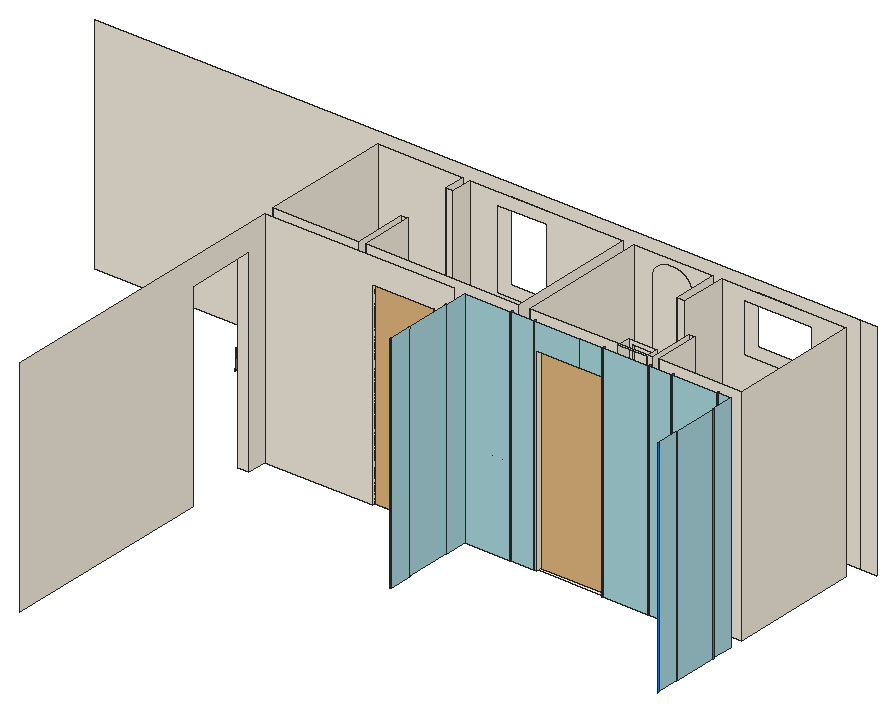
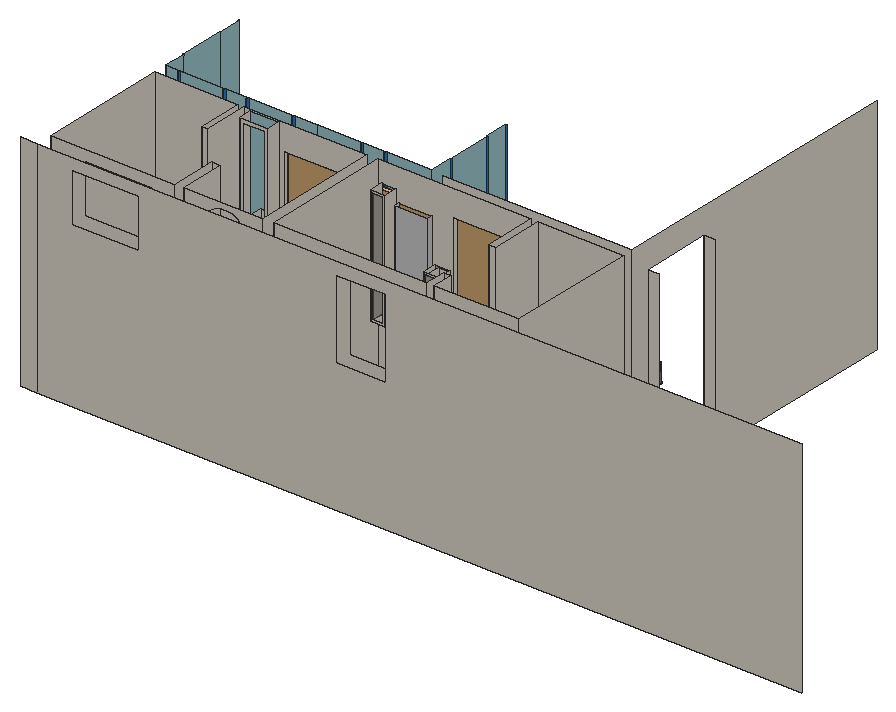
# SketchUp Ruby script. Lengths in inches.
U = 1.inch
M = Sketchup.active_model
def pt(a) = Geom::Point3d.new(a.map { |v| v * U })
def face(e, loops, mat)
  f = e.add_face(loops[0].map { |a| pt(a) })
  loops[1..].each { |l| e.add_face(l.map { |a| pt(a) }).erase! }
  f.material = f.back_material = mat if mat
  f
end
# faces: each face lists its corners as indices into pts; further lists are holes
def faces(e, pts, list, mat = nil) = list.each { |f| face(e, (f[0].is_a?(Array) ? f : [f]).map { |l| l.map { |i| pts[i] } }, mat) }
# xy, xz, yz: faces in a plane at the given z, y or x. An outline is a flat list of corners, or four numbers for a rectangle; further outlines are holes
def ring(l) = l.size == 4 ? [[l[0], l[1]], [l[2], l[1]], [l[2], l[3]], [l[0], l[3]]] : l.each_slice(2).to_a
def flat(e, list, mat, &to3) = list.each { |f| face(e, (f[0].is_a?(Array) ? f : [f]).map { |l| ring(l).map { |u, v| to3.(u, v) } }, mat) }
def xy(e, z, list, mat = nil) = flat(e, list, mat) { |x, y| [x, y, z] }
def xz(e, y, list, mat = nil) = flat(e, list, mat) { |x, z| [x, y, z] }
def yz(e, x, list, mat = nil) = flat(e, list, mat) { |y, z| [x, y, z] }
def lines(e, pts, list) = list.each { |a, b| e.add_line(pt(pts[a]), pt(pts[b])) }
# prism: a flat outline (further loops are holes) pulled along v
def prism(e, loops, v, mat = nil)
  f = face(e, loops, mat); d = Geom::Vector3d.new(v.map { |x| x * U })
  f.pushpull(f.normal.samedirection?(d) ? d.length : -d.length)
end
def box(e, o, s, mat = nil) = prism(e, [[o, [o[0] + s[0], o[1], o[2]], [o[0] + s[0], o[1] + s[1], o[2]], [o[0], o[1] + s[1], o[2]]]], [0, 0, s[2]], mat)
def at(x, y, z, deg = 0) = Geom::Transformation.translation(pt([x, y, z])) * Geom::Transformation.rotation(ORIGIN, Z_AXIS, deg.degrees)
def axes(o, x, y, z) = Geom::Transformation.new([*x, 0, *y, 0, *z, 0, *pt(o).to_a, 1])
def part(name) = M.definitions.add(name)
# library, detail: a bought-in or finely detailed component or shape, given as its bounding box
def library(name, o, s) = part(name).tap { |d| box(d.entities, o, s) }
def detail(e, o, s) = box(e.add_group.entities, o, s)
def put(e, d, t, mat = nil) = e.add_instance(d, t).tap { |i| i.material = mat if mat }
def group(e, t, mat = nil) = e.add_group.tap { |g| g.transformation = t; g.material = mat if mat }.entities
root = M.entities
M.materials.add("Material \#1").color = [140, 140, 140]
M.materials.add("[0030_OldLace]").color = [253, 245, 230]
M.materials.add("[0094_PowderBlue]").color = [176, 224, 230]
M.materials.add("[0098_DodgerBlue]").color = [30, 144, 255]
M.materials.add("[Granite Dark Gray]").color = [69, 68, 68]
M.materials.add("[Mirror 02]").color = [229, 229, 229]
M.materials.add("[Square Glass Tile 01]").color = [123, 142, 151]
M.materials.add("[Translucent Glass Gray]").color = [128, 128, 128]
M.materials["[Translucent Glass Gray]"].alpha = 0.5
c1 = library("door+(2)",[359.01,200.9,0],[123.81,2.27,104.69])
xy(root,0,[[302.04,512.67,335.61,533.42]])
xy(root,0,[[306.3125,459.46,341.0625,465.46]],"[0030_OldLace]")
xy(root,1.16,[[253.35,464.84,258.96,472.96]],"[0030_OldLace]")
xy(root,1.83,[[346.17,460.9,357.78,472.4]],"[0030_OldLace]")
xy(root,24.6,[[346.17,460.9,357.78,472.4]],"[0030_OldLace]")
xy(root,24.91,[[346.17,460.9,357.78,472.4]],"[0030_OldLace]")
xy(root,42.38,[[262.13,465.46,279.82,468.03]],"[0030_OldLace]")
xy(root,45.97,[[281.16,465.46,288.97,472.96]],"[0030_OldLace]")
xy(root,47.49,[[346.17,460.9,357.78,472.4]],"[0030_OldLace]")
xy(root,47.99,[[346.17,460.9,357.78,472.4]],"[0030_OldLace]")
xy(root,55.375,[[302.04,512.67,335.61,533.42]],"[Granite Dark Gray]")
xz(root,408.96,[[267,0,267.4375,120],[410.75,0,411,120]],"[0098_DodgerBlue]")
xz(root,409.46,[[410.75,0,411,120]],"[0098_DodgerBlue]")
xz(root,409.49,[[267,0,267.4375,120]],"[0098_DodgerBlue]")
xz(root,411.21,[[153,0,159,106]],"[0030_OldLace]")
xz(root,421.46,[[267,0,267.4375,120],[410.75,0,411,120]],"[0098_DodgerBlue]")
xz(root,421.96,[[267,0,267.4375,120],[410.75,0,411,120]],"[0098_DodgerBlue]")
xz(root,445.96,[[267,0,267.4375,120],[410.75,0,411,120]],"[0098_DodgerBlue]")
xz(root,446.46,[[267,0,267.4375,120],[410.75,0,411,120]],"[0098_DodgerBlue]")
xz(root,449.03,[[153,0,159,106]],"[0030_OldLace]")
xz(root,458.34,[[267.4375,0,292,120],[292.51,0,304.5,120],[305,0,306.3125,0,306.3125,106,329,106,329,120,305,120],[341.0625,0,341.5,0,341.5,120,329.5,120,329.5,106,341.0625,106],[342.01,0,366,120],
  [366.5,0,378.5,120],[379,0,402.99,120],[403.49,0,410.75,120]],"[0094_PowderBlue]")
xz(root,459.46,[[159,0,217.25,0,217.25,106,250.125,106,250.125,0,261,0,261,120,159,120]],"[0030_OldLace]")
xz(root,459.46,[[292,0,292.51,120],[304.5,0,305,120],[341.5,0,342.01,120],[366,0,366.5,120],[378.5,0,379,120],
  [402.99,0,403.49,120]],"[0098_DodgerBlue]")
xz(root,460.9,[[346.17,1.83,357.78,24.6],[346.17,24.91,357.78,47.49],[346.17,47.99,357.78,70.57]],"[0030_OldLace]")
xz(root,464.84,[[253.35,1.16,258.96,78.79]],"[0030_OldLace]")
xz(root,465.46,[[159,0,204.96,120],[[208.56,0,208.56,120,291,120,291,0,260.11,0,260.11,79.94,252.2,79.94,252.2,0,250.125,0,250.125,106,217.25,106,217.25,0],[262.13,42.38,279.82,102.76],[281.16,45.97,288.97,109.28]],[297,0,297,120,362.99,120,362.99,0,359.6,0,359.6,119.07,344.34,119.07,344.34,0,341.0625,0,341.0625,106,306.3125,106,306.3125,0],[366.13,0,411,120]],"[0030_OldLace]")
xz(root,468.03,[[262.13,42.38,279.82,102.76]],"[Mirror 02]")
xz(root,472.4,[[[344.34,0,359.6,119.07],[346.17,1.83,357.78,117.24]],[346.17,24.6,357.78,24.91],[346.17,47.49,357.78,47.99]],"[0030_OldLace]")
xz(root,472.4,[[346.17,1.83,357.78,24.6],[346.17,24.91,357.78,47.49],[346.17,47.99,357.78,70.57]],"[Translucent Glass Gray]")
xz(root,472.96,[[[252.2,0,260.11,79.94],[253.35,1.16,258.96,78.79]],[[281.16,45.97,288.97,109.28],[282.33,47.14,287.81,108.12]]],"[0030_OldLace]")
xz(root,472.96,[[253.35,1.16,258.96,78.79],[282.33,47.14,287.81,108.12]],"[Translucent Glass Gray]")
xz(root,489.9,[[362.99,0,366.13,120]],"[0030_OldLace]")
xz(root,493.9,[[204.96,0,208.56,120]],"[0030_OldLace]")
xz(root,511.15,[[339.125,0,343.94,120]],"[0030_OldLace]")
xz(root,512.67,[[302.04,0,335.61,55.375]],"[Granite Dark Gray]")
xz(root,524.21,[[204.96,0,208.56,120]],"[0030_OldLace]")
xz(root,533.42,[[302.04,0,335.61,55.375]])
xz(root,535.46,[[159,0,204.96,120],[[208.56,0,291,120],[223.25,70.875,250.125,113.5625]],[[297,0,339.125,120],[317.33,56.98,314.49,57.36,311.83,58.46,309.55,60.2,307.8,62.48,306.7,65.14,306.33,67.99,306.33,109.18,307.15,111.38,308.49,113.35,310.27,115,312.42,116.24,314.8125,117.01,317.33,117.27,319.86,117.01,322.25,116.24,324.39,115,326.18,113.35,327.52,111.38,328.34,109.18,328.34,67.99,327.96,65.14,326.86,62.48,325.12,60.2,322.84,58.46,320.18,57.36]],[[343.94,0,411,120],[356.125,87.625,392.375,114.125]]],"[0030_OldLace]")
xz(root,544.46,[[[0,0,411,120],[223.25,70.875,250.125,113.5625],[356.125,87.625,392.375,114.125]],[411,0,420,120]],"[0030_OldLace]")
yz(root,155.78,[[444.02,49.87,443.91,49.89,444.02,49.89],[444.02,49.87,444.02,49.89,444.13,49.9],[444.02,49.87,444.13,49.9,444.14,49.89],[443.91,49.89,443.91,49.9,444.02,49.89],[443.91,49.9,443.8,49.93,443.81,49.94],
  [443.8,49.93,443.71,49.99,443.81,49.94],[444.24,49.93,444.34,50,444.34,49.99],[443.81,49.94,443.71,49.99,443.71,50],[443.71,49.99,443.62,50.08,443.71,50],[444.34,49.99,444.34,50,444.42,50.09],
  [444.34,49.99,444.42,50.09,444.43,50.08],[444.43,50.08,444.42,50.09,444.49,50.19],[444.43,50.08,444.49,50.19,444.5,50.18],[443.99,50.11,443.95,50.125,443.99,50.125],[443.99,50.11,443.99,50.125,444.02,50.12],
  [443.99,50.11,444.02,50.12,444.02,50.11],[444.02,50.11,444.02,50.12,444.06,50.125],[444.02,50.11,444.06,50.125,444.0625,50.11],[444.0625,50.11,444.06,50.125,444.09,50.14],[444.0625,50.11,444.09,50.14,444.1,50.125],
  [443.95,50.125,443.92,50.15,443.95,50.14],[443.95,50.125,443.95,50.14,443.99,50.125],[444.5,50.18,444.49,50.19,444.56,50.31],[444.5,50.18,444.56,50.31,444.57,50.31],[444.18,50.21,444.19,50.26,444.2,50.25],
  [444.2,50.25,444.19,50.26,444.21,50.3],[444.2,50.25,444.21,50.3,444.22,50.3],[444.21,50.3,444.22,50.35,444.22,50.3],[444.22,50.3,444.22,50.35,444.23,50.35],[443.48,50.31,443.43,50.44,443.49,50.31],
  [443.49,50.31,443.43,50.44,443.44,50.45],[444.56,50.31,444.6,50.45,444.57,50.31],[444.57,50.31,444.6,50.45,444.61,50.44],[444.22,50.35,444.22,50.39,444.23,50.35],[444.23,50.35,444.22,50.39,444.23,50.39],
  [444.22,50.39,444.22,50.45,444.23,50.39],[444.23,50.39,444.22,50.45,444.23,50.45],[443.43,50.44,443.4,50.59,443.44,50.45],[443.44,50.45,443.4,50.59,443.41,50.59],[444.22,50.45,444.21,50.5,444.23,50.45],
  [444.23,50.45,444.21,50.5,444.22,50.5],[444.21,50.5,444.19,50.54,444.22,50.5],[444.22,50.5,444.19,50.54,444.2,50.55],[443.85,50.54,443.86,50.59,443.87,50.58],[444.19,50.54,444.17,50.58,444.2,50.55],
  [444.2,50.55,444.17,50.58,444.18,50.59],[443.87,50.58,443.86,50.59,443.89,50.62],[443.87,50.58,443.89,50.62,443.9,50.61],[444.17,50.58,444.15,50.61,444.18,50.59],[443.4,50.59,443.39,50.76,443.41,50.59],
  [444.18,50.59,444.15,50.61,444.16,50.62],[444.63,50.59,444.64,50.76,444.64,50.59],[444.64,50.59,444.64,50.76,444.65,50.76],[443.9,50.61,443.89,50.62,443.92,50.65],[443.9,50.61,443.92,50.65,443.92,50.64],
  [444.15,50.61,444.125,50.64,444.16,50.62],[444.16,50.62,444.125,50.64,444.13,50.65],[443.92,50.64,443.92,50.65,443.95,50.67],[443.92,50.64,443.95,50.67,443.95,50.66],[444.125,50.64,444.09,50.66,444.13,50.65],
  [443.95,50.66,443.95,50.67,443.99,50.6875],[443.95,50.66,443.99,50.6875,443.99,50.67],[444.64,50.76,444.64,60.79,444.65,50.76]],"Material \#1")
yz(root,159,[[295.46,0,411.21,0,411.21,106,449.03,106,449.03,0,459.46,0,459.46,120,295.46,120],[465.46,0,535.46,120]],"[0030_OldLace]")
yz(root,204.96,[[465.46,0,493.9,120],[524.21,0,535.46,120]],"[0030_OldLace]")
yz(root,208.56,[[465.46,0,493.9,120],[524.21,0,535.46,120]],"[0030_OldLace]")
yz(root,217.25,[[459.46,0,465.46,106]],"[0030_OldLace]")
yz(root,250.125,[[459.46,0,465.46,106]],"[0030_OldLace]")
yz(root,252.2,[[465.46,0,472.96,79.94]],"[0030_OldLace]")
yz(root,253.35,[[464.84,1.16,472.96,78.79]],"[0030_OldLace]")
yz(root,258.96,[[464.84,1.16,472.96,78.79]],"[0030_OldLace]")
yz(root,260.11,[[465.46,0,472.96,79.94]],"[0030_OldLace]")
yz(root,262.13,[[465.46,42.38,468.03,102.76]],"[Mirror 02]")
yz(root,267,[[408.96,0,409.49,120],[421.46,0,421.96,120],[445.96,0,446.46,120]],"[0098_DodgerBlue]")
yz(root,267.4375,[[409.49,0,421.46,120],[421.96,0,445.96,120],[446.46,0,458.34,120]],"[0094_PowderBlue]")
yz(root,279.82,[[465.46,42.38,468.03,102.76]],"[0030_OldLace]")
yz(root,281.16,[[465.46,45.97,472.96,109.28]],"[0030_OldLace]")
yz(root,288.97,[[465.46,45.97,472.96,109.28]],"[0030_OldLace]")
yz(root,291,[[465.46,0,535.46,120]],"[0030_OldLace]")
yz(root,292,[[458.34,0,459.46,120]],"[0098_DodgerBlue]")
yz(root,292.51,[[458.34,0,459.46,120]],"[0098_DodgerBlue]")
yz(root,297,[[465.46,0,535.46,120]],"[0030_OldLace]")
yz(root,302.04,[[512.67,0,533.42,55.375]],"[Granite Dark Gray]")
yz(root,304.5,[[458.34,0,459.46,120]],"[0098_DodgerBlue]")
yz(root,305,[[458.34,0,459.46,120]],"[0098_DodgerBlue]")
yz(root,306.3125,[[458.34,0,465.46,106]],"[0030_OldLace]")
yz(root,335.61,[[512.67,0,533.42,55.375]],"[Granite Dark Gray]")
yz(root,339.125,[[511.15,0,535.46,120]],"[0030_OldLace]")
yz(root,341.0625,[[458.34,0,465.46,106]],"[0030_OldLace]")
yz(root,341.5,[[458.34,0,459.46,120]],"[0098_DodgerBlue]")
yz(root,342.01,[[458.34,0,459.46,120]],"[0098_DodgerBlue]")
yz(root,343.94,[[511.15,0,535.46,120]],"[0030_OldLace]")
yz(root,344.34,[[465.46,0,472.4,119.07]],"[0030_OldLace]")
yz(root,346.17,[[460.9,1.83,472.4,24.6],[460.9,24.6,472.4,24.91],[460.9,24.91,472.4,47.49],[460.9,47.49,472.4,47.99],[460.9,47.99,472.4,70.57]],"[0030_OldLace]")
yz(root,357.78,[[460.9,1.83,472.4,24.6],[460.9,24.91,472.4,47.49],[460.9,47.99,472.4,70.57]],"[0030_OldLace]")
yz(root,359.6,[[465.46,0,472.4,119.07]],"[0030_OldLace]")
yz(root,362.99,[[465.46,0,489.9,120]],"[0030_OldLace]")
yz(root,366,[[458.34,0,459.46,120]],"[0098_DodgerBlue]")
yz(root,366.13,[[465.46,0,489.9,120]],"[0030_OldLace]")
yz(root,366.5,[[458.34,0,459.46,120]],"[0098_DodgerBlue]")
yz(root,378.5,[[458.34,0,459.46,120]],"[0098_DodgerBlue]")
yz(root,379,[[458.34,0,459.46,120]],"[0098_DodgerBlue]")
yz(root,402.99,[[458.34,0,459.46,120]],"[0098_DodgerBlue]")
yz(root,403.49,[[458.34,0,459.46,120]],"[0098_DodgerBlue]")
yz(root,410.75,[[409.46,0,421.46,120],[421.96,0,445.96,120],[446.46,0,458.34,120]],"[0094_PowderBlue]")
yz(root,411,[[465.46,0,535.46,120]],"[0030_OldLace]")
yz(root,411,[[408.96,0,409.46,120],[421.46,0,421.96,120],[445.96,0,446.46,120]],"[0098_DodgerBlue]")
p = [[282.33,472.96,47.14],[282.33,458.34,47.14],[287.81,472.96,47.14],[287.81,458.34,47.14]]
lines(root,p,[[0,1],[2,3]])
g1 = group(root,at(159,465.46,0),"[Square Glass Tile 01]")
xy(g1,0,[[0,0,132,70]])
put(root,c1,at(-141.76,260.21,0))
g2 = group(root,at(297,465.46,0),"[Square Glass Tile 01]")
xy(g2,0,[[0,0,114,70]])
